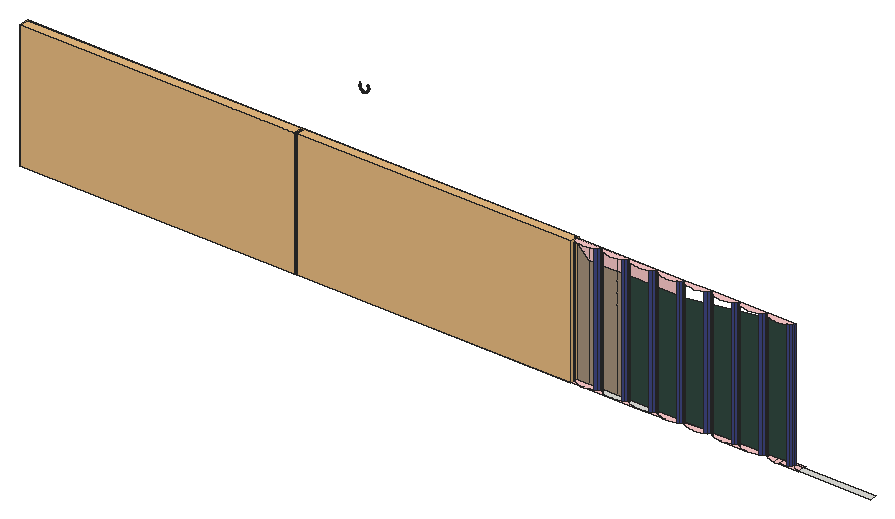
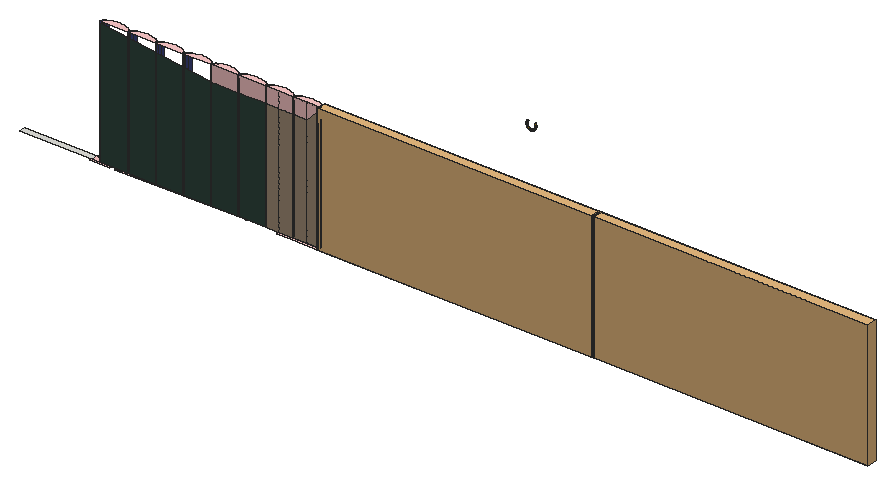
# SketchUp Ruby script. Lengths in inches.
U = 1.inch
M = Sketchup.active_model
def pt(a) = Geom::Point3d.new(a.map { |v| v * U })
def face(e, loops, mat)
  f = e.add_face(loops[0].map { |a| pt(a) })
  loops[1..].each { |l| e.add_face(l.map { |a| pt(a) }).erase! }
  f.material = f.back_material = mat if mat
  f
end
# faces: each face lists its corners as indices into pts; further lists are holes
def faces(e, pts, list, mat = nil) = list.each { |f| face(e, (f[0].is_a?(Array) ? f : [f]).map { |l| l.map { |i| pts[i] } }, mat) }
# xy, xz, yz: faces in a plane at the given z, y or x. An outline is a flat list of corners, or four numbers for a rectangle; further outlines are holes
def ring(l) = l.size == 4 ? [[l[0], l[1]], [l[2], l[1]], [l[2], l[3]], [l[0], l[3]]] : l.each_slice(2).to_a
def flat(e, list, mat, &to3) = list.each { |f| face(e, (f[0].is_a?(Array) ? f : [f]).map { |l| ring(l).map { |u, v| to3.(u, v) } }, mat) }
def xy(e, z, list, mat = nil) = flat(e, list, mat) { |x, y| [x, y, z] }
def xz(e, y, list, mat = nil) = flat(e, list, mat) { |x, z| [x, y, z] }
def yz(e, x, list, mat = nil) = flat(e, list, mat) { |y, z| [x, y, z] }
def lines(e, pts, list) = list.each { |a, b| e.add_line(pt(pts[a]), pt(pts[b])) }
# prism: a flat outline (further loops are holes) pulled along v
def prism(e, loops, v, mat = nil)
  f = face(e, loops, mat); d = Geom::Vector3d.new(v.map { |x| x * U })
  f.pushpull(f.normal.samedirection?(d) ? d.length : -d.length)
end
def box(e, o, s, mat = nil) = prism(e, [[o, [o[0] + s[0], o[1], o[2]], [o[0] + s[0], o[1] + s[1], o[2]], [o[0], o[1] + s[1], o[2]]]], [0, 0, s[2]], mat)
def at(x, y, z, deg = 0) = Geom::Transformation.translation(pt([x, y, z])) * Geom::Transformation.rotation(ORIGIN, Z_AXIS, deg.degrees)
def axes(o, x, y, z) = Geom::Transformation.new([*x, 0, *y, 0, *z, 0, *pt(o).to_a, 1])
def part(name) = M.definitions.add(name)
# library, detail: a bought-in or finely detailed component or shape, given as its bounding box
def library(name, o, s) = part(name).tap { |d| box(d.entities, o, s) }
def detail(e, o, s) = box(e.add_group.entities, o, s)
def put(e, d, t, mat = nil) = e.add_instance(d, t).tap { |i| i.material = mat if mat }
def group(e, t, mat = nil) = e.add_group.tap { |g| g.transformation = t; g.material = mat if mat }.entities
root = M.entities
M.materials.add("Generic").color = [169, 148, 125]
M.materials.add("Material \#68").color = [50, 74, 65]
M.materials.add("[0105_Navy]").color = [62, 69, 128]
M.materials.add("[0135_DarkGray]").color = [96, 79, 68]
M.materials.add("[Color A01]").color = [255, 204, 204]
M.materials.add("[Color D06]").color = [204, 153, 0]
c1 = library("Headwall panel",[0,-0.03,0],[4.39,126.03,32.28])
xy(root,46.28,[[183.46,751.11,183.68,751.11,183.91,751.12,184.54,751.15,185.56,751.33,186.46,751.63,187.17,752.05,187.64,752.53,187.84,753.07,187.82,753.18,179.55,753.18,179.57,753.07,179.62,752.75,179.98,752.24,180.59,751.79,181.41,751.4375,182.39,751.2],[191.73,751.11,191.95,751.11,192.18,751.12,192.81,751.15,193.83,751.33,194.73,751.63,195.43,752.05,195.9,752.53,196.1,753.07,196.09,753.18,193.19,753.18,187.84,753.07,187.88,752.75,188.24,752.24,188.86,751.79,189.68,751.4375,190.66,751.2],[234,751.14,234,753.18,234.15,751.15],[240,751.27,261.625,753.18],[215.02,753.18,219.4375,753.18,232.4375,754.01]])
xy(root,46.28,[[171.28,751.11,175.1,751.11,174.125,751.2,173.15,751.4375,172.32,751.79,171.71,752.24,171.35,752.75,171.28,753.18],[175.1,751.11,175.42,751.11,175.64,751.12,176.27,751.15,177.3,751.33,178.19,751.63,178.9,752.05,179.37,752.53,179.57,753.07,179.55,753.18,171.28,753.18,171.35,752.75,171.71,752.24,172.32,751.79,173.15,751.4375,174.125,751.2],[175.19,751.11,183.46,751.11,182.39,751.2,181.41,751.4375,180.59,751.79,179.98,752.24,179.62,752.75,179.57,753.07,179.37,752.53,178.9,752.05,178.19,751.63,177.3,751.33,176.27,751.15,175.64,751.12,175.42,751.11],[183.46,751.11,191.73,751.11,190.66,751.2,189.68,751.4375,188.86,751.79,188.24,752.24,187.88,752.75,187.84,753.07,187.64,752.53,187.17,752.05,186.46,751.63,185.56,751.33,184.54,751.15,183.91,751.12,183.68,751.11],[191.73,751.11,200,751.11,198.93,751.2,197.95,751.4375,197.125,751.79,196.51,752.24,196.15,752.75,196.1,753.07,195.9,752.53,195.43,752.05,194.73,751.63,193.83,751.33,192.81,751.15,192.18,751.12,191.95,751.11],
  [200,751.11,200.22,751.11,200.45,751.12,201.08,751.15,202.1,751.33,203,751.63,203.7,752.05,204.17,752.53,204.37,753.07,204.35,753.18,196.09,753.18,196.1,753.07,196.15,752.75,196.51,752.24,197.125,751.79,197.95,751.4375,198.93,751.2],[208.26,751.11,207.2,751.2,206.22,751.4375,205.39,751.79,204.78,752.24,204.42,752.75,214,753.18,215.02,753.18,212.64,753.07,212.44,752.53,211.97,752.05,211.26,751.63,210.37,751.33,209.35,751.15,208.71,751.12,208.49,751.11],[216.53,751.11,215.46,751.2,214.49,751.4375,213.66,751.79,213.05,752.24,212.6875,752.75,219.4375,753.18,222.29,753.18,220.91,753.07,220.71,752.53,220.24,752.05,219.53,751.63,218.64,751.33,217.61,751.15,216.98,751.12,216.76,751.11],[216.53,751.11,224.8,751.11,223.73,751.2,222.75,751.4375,221.93,751.79,221.32,752.24,220.96,752.75,220.91,753.07,220.71,752.53,220.24,752.05,219.53,751.63,218.64,751.33,217.61,751.15,216.98,751.12,216.76,751.11],[224.8,751.11,225.02,751.11,225.25,751.12,225.88,751.15,226.91,751.33,227.8,751.63,228.51,752.05,228.98,752.53,229.18,753.07,229.22,752.75,229.59,752.24,230.2,751.79,231.02,751.4375,232,751.2,232.4375,751.16,232.4375,753.18,222.29,753.18,220.91,753.07,220.96,752.75,221.32,752.24,221.93,751.79,222.75,751.4375,223.73,751.2],
  [233.07,751.11,233.29,751.11,233.52,751.12,234,751.14,234,753.18,232.4375,753.18,232.4375,751.16],[234,751.11,240,751.11,240,751.27,239.29,751.4375,238.47,751.79,237.85,752.24,237.49,752.75,237.44,753.07,237.24,752.53,236.78,752.05,236.07,751.63,235.17,751.33,234.15,751.15,234,751.14],[234.15,751.15,234,753.18,237.43,753.18,237.44,753.07,237.24,752.53,236.78,752.05,236.07,751.63,235.17,751.33],[240,751.27,240,753.18,237.43,753.18,237.44,753.07,237.49,752.75,237.85,752.24,238.47,751.79,239.29,751.4375],[204.42,752.75,214,753.18,204.35,753.18,204.37,753.07],
  [212.6875,752.75,212.64,753.07,215.02,753.18,219.4375,753.18],[171.28,753.18,171.28,753.5,171.26,753.41],[171.28,753.18,175.42,753.18,175.42,754.01,171.375,754.01,171.28,753.5],[175.42,753.18,179.55,753.18,179.53,753.41,179.49,754.01,175.42,754.01],[179.55,753.18,183.68,753.18,183.68,754.01,179.65,754.01,179.53,753.41],
  [193.19,753.18,232.4375,754.01,232.4375,753.18,222.29,753.18,232.4375,754.01,214,753.18],[214,753.18,232.4375,754.01,215.02,753.18],[219.4375,753.18,232.4375,754.01,222.29,753.18],[234,753.18,240,754.01]],"[Color A01]")
xy(root,84.3,[[175.19,751.11,174.125,751.2,173.15,751.4375,172.32,751.79,171.71,752.24,171.35,752.75,171.28,753.18,179.55,753.18,179.57,753.07,179.37,752.53,178.9,752.05,178.19,751.63,177.3,751.33,176.27,751.15,175.64,751.12,175.42,751.11],[183.46,751.11,182.39,751.2,181.41,751.4375,180.59,751.79,179.98,752.24,179.62,752.75,179.57,753.07,179.55,753.18,187.82,753.18,187.84,753.07,187.64,752.53,187.17,752.05,186.46,751.63,185.56,751.33,184.54,751.15,183.91,751.12,183.68,751.11],[191.73,751.11,190.66,751.2,189.68,751.4375,188.86,751.79,188.24,752.24,187.88,752.75,187.84,753.07,187.82,753.18,196.09,753.18,196.1,753.07,195.9,752.53,195.43,752.05,194.73,751.63,193.83,751.33,192.81,751.15,192.18,751.12,191.95,751.11],[200,751.11,198.93,751.2,197.95,751.4375,197.125,751.79,196.51,752.24,196.15,752.75,196.1,753.07,196.09,753.18,204.35,753.18,204.37,753.07,204.17,752.53,203.7,752.05,203,751.63,202.1,751.33,201.08,751.15,200.45,751.12,200.22,751.11],[208.26,751.11,207.2,751.2,206.22,751.4375,205.39,751.79,204.78,752.24,204.42,752.75,204.37,753.07,204.35,753.18,212.62,753.18,212.64,753.07,212.44,752.53,211.97,752.05,211.26,751.63,210.37,751.33,209.35,751.15,208.71,751.12,208.49,751.11],
  [216.53,751.11,215.46,751.2,214.49,751.4375,213.66,751.79,213.05,752.24,212.6875,752.75,212.64,753.07,212.62,753.18,220.89,753.18,220.91,753.07,220.71,752.53,220.24,752.05,219.53,751.63,218.64,751.33,217.61,751.15,216.98,751.12,216.76,751.11],[224.8,751.11,223.73,751.2,222.75,751.4375,221.93,751.79,221.32,752.24,220.96,752.75,220.91,753.07,220.89,753.18,229.16,753.18,229.18,753.07,228.98,752.53,228.51,752.05,227.8,751.63,226.91,751.33,225.88,751.15,225.25,751.12,225.02,751.11],[233.07,751.11,232,751.2,231.02,751.4375,230.2,751.79,229.59,752.24,229.22,752.75,229.18,753.07,229.16,753.18,237.43,753.18,237.44,753.07,237.24,752.53,236.78,752.05,236.07,751.63,235.17,751.33,234.15,751.15,233.52,751.12,233.29,751.11]],"[Color A01]")
xz(root,753.18,[[171.28,46.28,175.42,46.28,175.42,79.63,171.28,83.97],[175.42,46.28,179.55,79.63],[179.55,46.28,183.68,79.63],[183.68,46.28,187.82,79.63]],"Generic")
xz(root,753.18,[[187.82,46.28,196.09,79.63],[196.09,46.28,204.35,79.63],[204.35,46.28,237.43,46.28,237.43,83.97,204.35,79.63]],"Material \#68")
xz(root,753.18,[[175.42,79.63,175.42,84.3,171.28,84.3,171.28,83.97],[175.42,79.63,179.55,84.3],[179.55,79.63,183.68,84.3],[183.68,79.63,187.82,84.3],[187.82,79.63,196.09,84.3],
  [196.09,79.63,204.35,84.3]],"[Color A01]")
xz(root,753.58,[[107.55,100.6,107.55,100.99,107.43,101,107.39,100.61],[107.55,100.6,107.71,100.61,107.67,101,107.55,100.99],[107.39,100.61,107.43,101,107.3125,101.02,107.23,100.63],[107.71,100.61,107.87,100.63,107.79,101.02,107.67,101],[107.23,100.63,107.3125,101.02,107.2,101.05,107.08,100.68],
  [107.87,100.63,108.03,100.68,107.9,101.05,107.79,101.02],[107.08,100.68,107.2,101.05,107.09,101.09,106.93,100.73],[108.03,100.68,108.18,100.73,108.02,101.09,107.9,101.05],[106.93,100.73,107.09,101.09,106.98,101.15,106.78,100.81],[108.18,100.73,108.32,100.81,108.12,101.15,108.02,101.09],
  [106.78,100.81,106.98,101.15,106.88,101.21,106.65,100.89],[108.32,100.81,108.45,100.89,108.22,101.21,108.12,101.15],[106.65,100.89,106.88,101.21,106.79,101.29,106.52,101],[108.45,100.89,108.58,101,108.32,101.29,108.22,101.21],[106.52,101,106.79,101.29,106.7,101.375,106.41,101.11],
  [108.58,101,108.69,101.11,108.4,101.375,108.32,101.29],[106.41,101.11,106.7,101.375,106.625,101.47,106.31,101.23],[108.69,101.11,108.79,101.23,108.48,101.47,108.4,101.375],[106.31,101.23,106.625,101.47,106.56,101.57,106.22,101.37],[108.79,101.23,108.88,101.37,108.54,101.57,108.48,101.47],
  [106.22,101.37,106.56,101.57,106.51,101.67,106.15,101.51],[108.88,101.37,108.95,101.51,108.59,101.67,108.54,101.57],[106.15,101.51,106.51,101.67,106.46,101.78,106.09,101.66],[108.95,101.51,109.01,101.66,108.64,101.78,108.59,101.67],[106.09,101.66,106.46,101.78,106.43,101.9,106.05,101.82],
  [109.01,101.66,109.05,101.82,108.67,101.9,108.64,101.78],[106.05,101.82,106.43,101.9,106.41,102.02,106.02,101.98],[109.05,101.82,109.08,101.98,108.6875,102.02,108.67,101.9],[106.02,101.98,106.41,102.02,106.41,102.14,106.01,102.14],[109.08,101.98,109.09,102.14,108.69,102.14,108.6875,102.02],
  [106.01,102.14,106.41,102.14,106.41,102.26,106.02,102.3],[108.69,102.14,109.09,102.14,109.08,102.3,108.6875,102.26],[106.41,102.26,106.43,102.375,106.05,102.46,106.02,102.3],[108.6875,102.26,109.08,102.3,109.05,102.46,108.67,102.375],[106.43,102.375,106.46,102.49,106.09,102.61,106.05,102.46],
  [108.67,102.375,109.05,102.46,109.01,102.61,108.64,102.49],[106.46,102.49,106.51,102.6,106.15,102.76,106.09,102.61],[108.64,102.49,109.01,102.61,108.95,102.76,108.59,102.6],[106.51,102.6,106.56,102.71,106.22,102.91,106.15,102.76],[108.59,102.6,108.95,102.76,108.88,102.91,108.54,102.71],
  [106.56,102.71,106.625,102.81,106.31,103.04,106.22,102.91],[108.54,102.71,108.88,102.91,108.79,103.04,108.48,102.81],[108.48,102.81,108.79,103.04,108.69,103.17,108.4,102.9]],"[Color D06]")
yz(root,171.28,[[753.18,46.28,753.18,83.97,754.01,79.63,754.01,46.28]],"Material \#68")
p = [[178.9,752.05,46.28],[178.19,751.63,46.28],[178.19,751.63,84.3],[178.9,752.05,84.3],[187.17,752.05,46.28],[186.46,751.63,46.28],
  [186.46,751.63,84.3],[187.17,752.05,84.3],[195.43,752.05,46.28],[194.73,751.63,46.28],[194.73,751.63,84.3],[195.43,752.05,84.3],
  [203.7,752.05,46.28],[203,751.63,46.28],[203,751.63,84.3],[203.7,752.05,84.3],[211.97,752.05,46.28],[211.26,751.63,46.28],
  [211.26,751.63,84.3],[211.97,752.05,84.3],[220.24,752.05,46.28],[219.53,751.63,46.28],[219.53,751.63,84.3],[220.24,752.05,84.3],
  [228.51,752.05,46.28],[227.8,751.63,46.28],[227.8,751.63,84.3],[228.51,752.05,84.3],[236.78,752.05,46.28],[236.07,751.63,46.28],
  [236.07,751.63,84.3],[236.78,752.05,84.3],[172.32,751.79,46.28],[171.71,752.24,46.28],[171.71,752.24,84.3],[172.32,751.79,84.3],
  [180.59,751.79,46.28],[179.98,752.24,46.28],[179.98,752.24,84.3],[180.59,751.79,84.3],[188.86,751.79,46.28],[188.24,752.24,46.28],
  [188.24,752.24,84.3],[188.86,751.79,84.3],[197.125,751.79,46.28],[196.51,752.24,46.28],[196.51,752.24,84.3],[197.125,751.79,84.3],
  [205.39,751.79,46.28],[204.78,752.24,46.28],[204.78,752.24,84.3],[205.39,751.79,84.3],[213.66,751.79,46.28],[213.05,752.24,46.28],
  [213.05,752.24,84.3],[213.66,751.79,84.3],[221.93,751.79,46.28],[221.32,752.24,46.28],[221.32,752.24,84.3],[221.93,751.79,84.3],
  [230.2,751.79,46.28],[229.59,752.24,46.28],[229.59,752.24,84.3],[230.2,751.79,84.3],[179.37,752.53,46.28],[179.37,752.53,84.3],
  [187.64,752.53,46.28],[187.64,752.53,84.3],[195.9,752.53,46.28],[195.9,752.53,84.3],[204.17,752.53,46.28],[204.17,752.53,84.3],
  [212.44,752.53,46.28],[212.44,752.53,84.3],[220.71,752.53,46.28],[220.71,752.53,84.3],[228.98,752.53,46.28],[228.98,752.53,84.3],
  [237.24,752.53,46.28],[237.24,752.53,84.3],[171.35,752.75,46.28],[171.35,752.75,84.3],[179.62,752.75,46.28],[179.62,752.75,84.3],
  [187.88,752.75,46.28],[187.88,752.75,84.3],[196.15,752.75,46.28],[196.15,752.75,84.3],[204.42,752.75,46.28],[204.42,752.75,84.3],
  [212.6875,752.75,46.28],[212.6875,752.75,84.3],[220.96,752.75,46.28],[220.96,752.75,84.3],[229.22,752.75,46.28],[229.22,752.75,84.3],
  [179.57,753.07,46.28],[179.57,753.07,84.3],[187.84,753.07,46.28],[187.84,753.07,84.3],[196.1,753.07,46.28],[196.1,753.07,84.3],
  [204.37,753.07,46.28],[204.37,753.07,84.3],[212.64,753.07,46.28],[212.64,753.07,84.3],[220.91,753.07,46.28],[220.91,753.07,84.3],
  [229.18,753.07,46.28],[229.18,753.07,84.3],[237.44,753.07,46.28],[237.44,753.07,84.3],[171.28,753.18,46.28],[171.28,753.18,83.97],
  [171.28,753.18,84.3],[179.55,753.18,46.28],[179.55,753.18,79.63],[179.55,753.18,84.3],[187.82,753.18,46.28],[187.82,753.18,79.63],
  [187.82,753.18,84.3],[196.09,753.18,46.28],[196.09,753.18,79.63],[196.09,753.18,84.3],[204.35,753.18,46.28],[204.35,753.18,79.63],
  [204.35,753.18,84.3],[237.43,753.18,46.28],[237.43,753.18,84.3],[237.43,753.18,83.97],[237.85,752.24,79.93],[238.47,751.79,79.93],
  [245.04,752.05,46.28],[245.51,752.53,46.28],[237.49,752.75,79.93]]
faces(root,p,[[0,1,2,3],[4,5,6,7],[8,9,10,11],[12,13,14,15],[16,17,18,19],[20,21,22,23],[24,25,26,27],[28,29,30,31],
  [32,33,34,35],[36,37,38,39],[40,41,42,43],[44,45,46,47],[48,49,50,51],[52,53,54,55],[56,57,58,59],[60,61,62,63],
  [64,0,3,65],[66,4,7,67],[68,8,11,69],[70,12,15,71],[72,16,19,73],[74,20,23,75],[76,24,27,77],[78,28,31,79],
  [33,80,81,34],[37,82,83,38],[41,84,85,42],[45,86,87,46],[49,88,89,50],[53,90,91,54],[57,92,93,58],[61,94,95,62],
  [96,64,65,97],[98,66,67,99],[100,68,69,101],[102,70,71,103],[104,72,73,105],[106,74,75,107],[108,76,77,109],[110,78,79,111],
  [80,112,113,114,81],[97,83,82,96],[99,85,84,98],[101,87,86,100],[103,89,88,102],[105,91,90,104],[107,93,92,106],[109,95,94,108],
  [127,110,111,128,129]],"[0105_Navy]")
faces(root,p,[[96,115,116,117,97],[98,118,119,120,99],[100,121,122,123,101],[102,124,125,126,103]],"[Color A01]")
lines(root,p,[[130,131],[132,133],[134,130],[111,134]])
put(root,c1,axes([5.99,754.01,46.28],[0,-0.66,0],[0.66,0,0],[0,0,1.17778]),"[0135_DarkGray]")
put(root,c1,axes([88.58,754.01,46.28],[0,-0.66,0],[0.66,0,0],[0,0,1.17778]),"[0105_Navy]")
